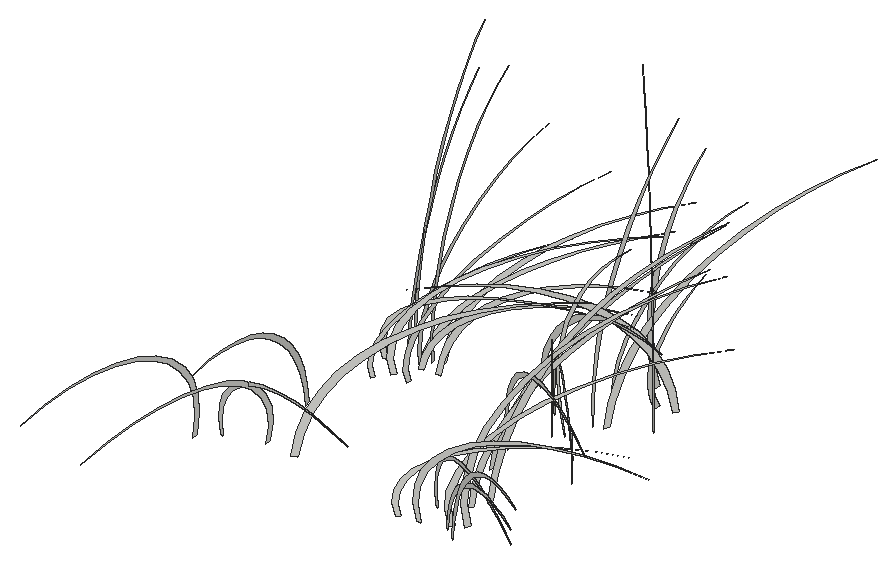
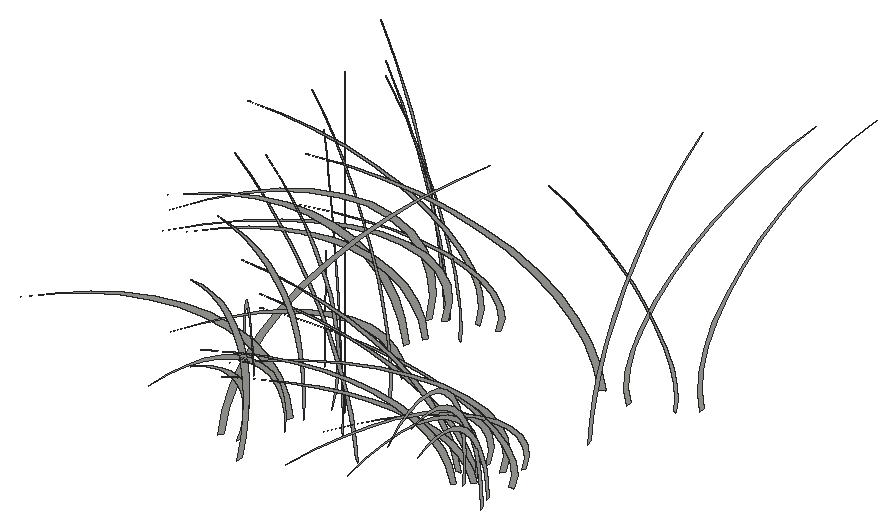
# SketchUp Ruby script. Lengths in inches.
U = 1.inch
M = Sketchup.active_model
def pt(a) = Geom::Point3d.new(a.map { |v| v * U })
def face(e, loops, mat)
  f = e.add_face(loops[0].map { |a| pt(a) })
  loops[1..].each { |l| e.add_face(l.map { |a| pt(a) }).erase! }
  f.material = f.back_material = mat if mat
  f
end
# faces: each face lists its corners as indices into pts; further lists are holes
def faces(e, pts, list, mat = nil) = list.each { |f| face(e, (f[0].is_a?(Array) ? f : [f]).map { |l| l.map { |i| pts[i] } }, mat) }
# xy, xz, yz: faces in a plane at the given z, y or x. An outline is a flat list of corners, or four numbers for a rectangle; further outlines are holes
def ring(l) = l.size == 4 ? [[l[0], l[1]], [l[2], l[1]], [l[2], l[3]], [l[0], l[3]]] : l.each_slice(2).to_a
def flat(e, list, mat, &to3) = list.each { |f| face(e, (f[0].is_a?(Array) ? f : [f]).map { |l| ring(l).map { |u, v| to3.(u, v) } }, mat) }
def xy(e, z, list, mat = nil) = flat(e, list, mat) { |x, y| [x, y, z] }
def xz(e, y, list, mat = nil) = flat(e, list, mat) { |x, z| [x, y, z] }
def yz(e, x, list, mat = nil) = flat(e, list, mat) { |y, z| [x, y, z] }
def lines(e, pts, list) = list.each { |a, b| e.add_line(pt(pts[a]), pt(pts[b])) }
# prism: a flat outline (further loops are holes) pulled along v
def prism(e, loops, v, mat = nil)
  f = face(e, loops, mat); d = Geom::Vector3d.new(v.map { |x| x * U })
  f.pushpull(f.normal.samedirection?(d) ? d.length : -d.length)
end
def box(e, o, s, mat = nil) = prism(e, [[o, [o[0] + s[0], o[1], o[2]], [o[0] + s[0], o[1] + s[1], o[2]], [o[0], o[1] + s[1], o[2]]]], [0, 0, s[2]], mat)
def at(x, y, z, deg = 0) = Geom::Transformation.translation(pt([x, y, z])) * Geom::Transformation.rotation(ORIGIN, Z_AXIS, deg.degrees)
def axes(o, x, y, z) = Geom::Transformation.new([*x, 0, *y, 0, *z, 0, *pt(o).to_a, 1])
def part(name) = M.definitions.add(name)
# library, detail: a bought-in or finely detailed component or shape, given as its bounding box
def library(name, o, s) = part(name).tap { |d| box(d.entities, o, s) }
def detail(e, o, s) = box(e.add_group.entities, o, s)
def put(e, d, t, mat = nil) = e.add_instance(d, t).tap { |i| i.material = mat if mat }
def group(e, t, mat = nil) = e.add_group.tap { |g| g.transformation = t; g.material = mat if mat }.entities
root = M.entities
g1 = group(root,at(13.87,756.7,-58.625))
p = [[0.42,-0.1875,0],[0.1875,-0.08,0],[0,0,0.76],[0.08,-0.03,1.52],[0.41,-0.18,2.27],[1,-0.45,2.98],
  [1.83,-0.82,3.65],[2.88,-1.28,4.24],[4.125,-1.84,4.76],[5.52,-2.46,5.17],[7.05,-3.14,5.49],[8.67,-3.86,5.6875],
  [10.34,-4.61,5.77],[12.01,-5.35,5.73],[10.37,-4.62,5.74],[8.74,-3.9,5.63],[7.17,-3.2,5.41],[5.69,-2.54,5.09],
  [4.33,-1.93,4.67],[3.13,-1.4,4.16],[2.11,-0.94,3.57],[1.3,-0.58,2.92],[0.72,-0.32,2.22],[0.37,-0.17,1.49],
  [0.27,-0.12,0.74]]
faces(g1,p,[[0,1,2,3,4,5,6,7,8,9,10,11,12,13,14,15,16,17,18,19,20,21,22,23,24]])
g2 = group(root,at(16.26,757.76,-58.625))
p = [[0.08,-0.6,0],[0.03,-0.27,0],[0,0,0.91],[0.01,-0.11,1.82],[0.07,-0.59,2.72],[0.18,-1.43,3.57],
  [0.33,-2.61,4.37],[0.52,-4.1,5.08],[0.74,-5.86,5.69],[0.99,-7.86,6.19],[1.26,-10.03,6.57],[1.55,-12.33,6.81],
  [1.85,-14.7,6.91],[2.15,-17.08,6.86],[1.86,-14.74,6.87],[1.57,-12.43,6.74],[1.28,-10.2,6.48],[1.02,-8.09,6.09],
  [0.78,-6.16,5.59],[0.5625,-4.45,4.98],[0.38,-3.01,4.28],[0.23,-1.85,3.5],[0.13,-1.02,2.66],[0.07,-0.53,1.79],
  [0.05,-0.39,0.89]]
faces(g2,p,[[0,1,2,3,4,5,6,7,8,9,10,11,12,13,14,15,16,17,18,19,20,21,22,23,24]])
g3 = group(root,at(17.87,768.3125,-58.625))
p = [[7.42,7.33,7.7],[8.54,8.44,7.91],[7.45,7.37,7.66],[6.41,6.33,7.32],[5.41,5.35,6.89],[4.47,4.42,6.37],
  [3.6,3.5625,5.77],[2.81,2.78,5.1],[2.12,2.09,4.37],[1.51,1.5,3.57],[1.02,1.01,2.73],[0.63,0.62,1.84],
  [0.35,0.35,0.93],[0.19,0.19,0],[0,0,0],[0.13,0.13,0.95],[0.39,0.38,1.89],[0.77,0.76,2.79],
  [1.27,1.26,3.66],[1.89,1.87,4.47],[2.61,2.58,5.21],[3.42,3.38,5.89],[4.32,4.27,6.48],[5.3,5.24,6.99],
  [6.33,6.26,7.39]]
faces(g3,p,[[0,1,2,3,4,5,6,7,8,9,10,11,12,13,14,15,16,17,18,19,20,21,22,23,24]])
g4 = group(root,at(17.79,765.61,-58.625))
p = [[0.04,0.5,0],[0.02,0.22,0],[0,0,0.75],[0.01,0.09,1.5],[0.04,0.49,2.24],[0.1,1.18,2.94],
  [0.17,2.16,3.59],[0.27,3.39,4.18],[0.39,4.85,4.6875],[0.53,6.5,5.1],[0.67,8.29,5.41],[0.82,10.19,5.6],
  [0.98,12.15,5.68],[1.14,14.12,5.64],[0.99,12.19,5.65],[0.83,10.28,5.55],[0.68,8.43,5.33],[0.54,6.69,5.02],
  [0.41,5.1,4.6],[0.3,3.68,4.1],[0.2,2.49,3.52],[0.125,1.53,2.88],[0.07,0.84,2.19],[0.04,0.4375,1.47],
  [0.03,0.32,0.73]]
faces(g4,p,[[0,1,2,3,4,5,6,7,8,9,10,11,12,13,14,15,16,17,18,19,20,21,22,23,24]])
g5 = group(root,at(16.61,765.86,-58.625))
p = [[0.33,0.33,0],[0.15,0.15,0],[0,0,0.88],[0.06,0.06,1.76],[0.32,0.32,2.63],[0.79,0.78,3.46],
  [1.43,1.42,4.23],[2.25,2.23,4.92],[3.22,3.1875,5.51],[4.32,4.27,6],[5.51,5.45,6.36],[6.77,6.7,6.59],
  [8.08,7.99,6.6875],[9.38,9.28,6.64],[8.1,8.01,6.65],[6.83,6.75,6.53],[5.6,5.54,6.28],[4.45,4.4,5.9],
  [3.39,3.35,5.41],[2.45,2.42,4.82],[1.65,1.63,4.14],[1.02,1.01,3.39],[0.5625,0.56,2.58],[0.29,0.29,1.73],
  [0.21,0.21,0.86]]
faces(g5,p,[[0,1,2,3,4,5,6,7,8,9,10,11,12,13,14,15,16,17,18,19,20,21,22,23,24]])
g6 = group(root,at(17.18,767.63,-58.625))
p = [[7.42,7.33,6.21],[8.54,8.44,6.375],[7.45,7.37,6.18],[6.41,6.33,5.9],[5.41,5.35,5.56],[4.47,4.42,5.14],
  [3.6,3.5625,4.66],[2.81,2.78,4.11],[2.12,2.09,3.52],[1.51,1.5,2.88],[1.02,1.01,2.2],[0.63,0.62,1.49],
  [0.35,0.35,0.75],[0.19,0.19,0],[0,0,0],[0.13,0.13,0.77],[0.39,0.38,1.52],[0.77,0.76,2.25],
  [1.27,1.26,2.95],[1.89,1.87,3.6],[2.61,2.58,4.21],[3.42,3.38,4.75],[4.32,4.27,5.23],[5.3,5.24,5.63],
  [6.33,6.26,5.96]]
faces(g6,p,[[0,1,2,3,4,5,6,7,8,9,10,11,12,13,14,15,16,17,18,19,20,21,22,23,24]])
g7 = group(root,at(27.74,768.2,-58.625))
p = [[4.83,11.72,10.21],[5.56,13.49,10.48],[4.85,11.77,10.15],[4.17,10.12,9.7],[3.52,8.54,9.13],[2.91,7.0625,8.44],
  [2.35,5.69,7.65],[1.83,4.45,6.76],[1.38,3.34,5.78],[0.99,2.39,4.73],[0.66,1.61,3.61],[0.41,0.99,2.44],
  [0.23,0.56,1.23],[0.125,0.31,0],[0,0,0],[0.09,0.21,1.26],[0.25,0.61,2.5],[0.5,1.22,3.7],
  [0.83,2.01,4.85],[1.23,2.98,5.92],[1.7,4.12,6.91],[2.23,5.4,7.8],[2.8125,6.83,8.59],[3.45,8.37,9.26],
  [4.125,10,9.8]]
faces(g7,p,[[0,1,2,3,4,5,6,7,8,9,10,11,12,13,14,15,16,17,18,19,20,21,22,23,24]])
g8 = group(root,at(26.19,755.85,-58.625))
p = [[0.5,0,0],[0.22,0,0],[0,0,0.95],[0.09,0,1.9],[0.49,0,2.83],[1.1875,-0.01,3.72],
  [2.17,-0.01,4.55],[3.41,-0.02,5.29],[4.87,-0.03,5.93],[6.53,-0.04,6.45],[8.33,-0.05,6.84],[10.24,-0.06,7.09],
  [12.21,-0.07,7.1875],[14.19,-0.08,7.14],[12.25,-0.07,7.15],[10.33,-0.06,7.02],[8.47,-0.05,6.75],[6.72,-0.04,6.35],
  [5.12,-0.03,5.82],[3.7,-0.02,5.18],[2.5,-0.01,4.45],[1.54,-0.01,3.64],[0.85,0,2.77],[0.44,0,1.86],
  [0.32,0,0.93]]
faces(g8,p,[[0,1,2,3,4,5,6,7,8,9,10,11,12,13,14,15,16,17,18,19,20,21,22,23,24]])
g9 = group(root,at(17.96,757.02,-58.625))
p = [[11.7,4.87,10.21],[13.47,5.61,10.48],[11.76,4.89,10.15],[10.11,4.21,9.7],[8.53,3.55,9.13],[7.05,2.94,8.44],
  [5.68,2.37,7.65],[4.44,1.85,6.76],[3.34,1.39,5.78],[2.39,0.99,4.73],[1.6,0.67,3.61],[0.99,0.41,2.44],
  [0.56,0.23,1.23],[0.3,0.125,0],[0,0,0],[0.21,0.09,1.26],[0.61,0.26,2.5],[1.22,0.51,3.7],
  [2.01,0.84,4.85],[2.98,1.24,5.92],[4.11,1.71,6.91],[5.4,2.25,7.8],[6.82,2.84,8.59],[8.36,3.48,9.26],
  [9.99,4.16,9.8]]
faces(g9,p,[[0,1,2,3,4,5,6,7,8,9,10,11,12,13,14,15,16,17,18,19,20,21,22,23,24]])
g10 = group(root,at(15.5,769.27,-58.625))
p = [[-4.01,9.63,10.42],[-4.61,11.08,10.69],[-4.03,9.68,10.36],[-3.46,8.32,9.9],[-2.92,7.02,9.32],[-2.42,5.8,8.62],
  [-1.95,4.68,7.81],[-1.52,3.65,6.9],[-1.14,2.75,5.9],[-0.82,1.97,4.83],[-0.55,1.32,3.6875],[-0.34,0.81,2.49],
  [-0.19,0.46,1.26],[-0.1,0.25,0],[0,0,0],[-0.07,0.17,1.29],[-0.21,0.5,2.55],[-0.42,1,3.78],
  [-0.6875,1.65,4.95],[-1.02,2.45,6.04],[-1.41,3.38,7.05],[-1.85,4.44,7.96],[-2.34,5.61,8.76],[-2.86,6.875,9.45],
  [-3.42,8.22,10]]
faces(g10,p,[[0,1,2,3,4,5,6,7,8,9,10,11,12,13,14,15,16,17,18,19,20,21,22,23,24]])
g11 = group(root,at(17.67,767.86,-58.625))
p = [[-0.18,0.43,0],[-0.08,0.19,0],[0,0,1.1875],[-0.03,0.08,2.38],[-0.17,0.42,3.56],[-0.42,1.02,4.68],
  [-0.77,1.86,5.72],[-1.22,2.92,6.65],[-1.74,4.18,7.45],[-2.33,5.6,8.11],[-2.98,7.16,8.6],[-3.66,8.8,8.91],
  [-4.36,10.49,9.04],[-5.07,12.18,8.98],[-4.38,10.52,8.99],[-3.69,8.87,8.83],[-3.03,7.28,8.49],[-2.4,5.77,7.98],
  [-1.83,4.4,7.32],[-1.32,3.18,6.52],[-0.89,2.15,5.6],[-0.55,1.32,4.58],[-0.3,0.73,3.48],[-0.16,0.38,2.34],
  [-0.12,0.28,1.17]]
faces(g11,p,[[0,1,2,3,4,5,6,7,8,9,10,11,12,13,14,15,16,17,18,19,20,21,22,23,24]])
g12 = group(root,at(17.43,767.15,-58.625))
p = [[-0.09,0.46,0],[-0.04,0.2,0],[0,0,0.88],[-0.02,0.08,1.76],[-0.09,0.45,2.63],[-0.21,1.08,3.46],
  [-0.38,1.98,4.23],[-0.6,3.11,4.92],[-0.86,4.45,5.51],[-1.16,5.96,6],[-1.48,7.61,6.36],[-1.8125,9.35,6.59],
  [-2.16,11.15,6.6875],[-2.51,12.96,6.64],[-2.17,11.18,6.65],[-1.83,9.43,6.53],[-1.5,7.74,6.28],[-1.19,6.14,5.9],
  [-0.91,4.67,5.41],[-0.66,3.38,4.82],[-0.44,2.28,4.14],[-0.27,1.41,3.39],[-0.15,0.77,2.58],[-0.08,0.4,1.73],
  [-0.06,0.29,0.86]]
faces(g12,p,[[0,1,2,3,4,5,6,7,8,9,10,11,12,13,14,15,16,17,18,19,20,21,22,23,24]])
g13 = group(root,at(15.87,768.38,-58.625))
p = [[-4.01,9.63,8.4],[-4.61,11.08,8.62],[-4.03,9.68,8.35],[-3.46,8.32,7.98],[-2.92,7.02,7.51],[-2.42,5.8,6.95],
  [-1.95,4.68,6.3],[-1.52,3.65,5.5625],[-1.14,2.75,4.76],[-0.82,1.97,3.89],[-0.55,1.32,2.97],[-0.34,0.81,2.01],
  [-0.19,0.46,1.02],[-0.1,0.25,0],[0,0,0],[-0.07,0.17,1.04],[-0.21,0.5,2.06],[-0.42,1,3.05],
  [-0.6875,1.65,3.99],[-1.02,2.45,4.87],[-1.41,3.38,5.6875],[-1.85,4.44,6.42],[-2.34,5.61,7.07],[-2.86,6.875,7.62],
  [-3.42,8.22,8.0625]]
faces(g13,p,[[0,1,2,3,4,5,6,7,8,9,10,11,12,13,14,15,16,17,18,19,20,21,22,23,24]])
g14 = group(root,at(25.05,764.17,-58.625))
p = [[0.45,-0.35,0],[0.2,-0.15,0],[0,0,1.07],[0.08,-0.0625,2.14],[0.4375,-0.34,3.2],[1.06,-0.82,4.2],
  [1.94,-1.5,5.14],[3.04,-2.36,5.98],[4.35,-3.375,6.7],[5.83,-4.52,7.29],[7.4375,-5.77,7.73],[9.14,-7.1,8.01],
  [10.9,-8.46,8.125],[12.67,-9.83,8.07],[10.93,-8.49,8.08],[9.22,-7.16,7.93],[7.5625,-5.87,7.625],[6,-4.66,7.17],
  [4.57,-3.55,6.58],[3.3,-2.56,5.86],[2.23,-1.73,5.03],[1.375,-1.07,4.12],[0.76,-0.59,3.13],[0.39,-0.3,2.1],
  [0.29,-0.22,1.05]]
faces(g14,p,[[0,1,2,3,4,5,6,7,8,9,10,11,12,13,14,15,16,17,18,19,20,21,22,23,24]])
g15 = group(root,at(22.73,769.59,-58.625))
p = [[11.19,-5.95,8.88],[12.88,-6.85,9.11],[11.24,-5.98,8.83],[9.66,-5.14,8.4375],[8.16,-4.34,7.94],[6.74,-3.59,7.34],
  [5.43,-2.89,6.66],[4.25,-2.26,5.88],[3.19,-1.7,5.03],[2.29,-1.22,4.12],[1.53,-0.82,3.14],[0.95,-0.5,2.125],
  [0.53,-0.28,1.07],[0.29,-0.16,0],[0,0,0],[0.2,-0.1,1.1],[0.59,-0.3125,2.18],[1.16,-0.62,3.22],
  [1.92,-1.02,4.22],[2.85,-1.51,5.15],[3.93,-2.09,6.01],[5.16,-2.74,6.79],[6.52,-3.47,7.47],[7.99,-4.25,8.05],
  [9.55,-5.08,8.52]]
faces(g15,p,[[0,1,2,3,4,5,6,7,8,9,10,11,12,13,14,15,16,17,18,19,20,21,22,23,24]])
g16 = group(root,at(27.9375,759.28,-58.625))
p = [[4.27,10.37,11.2],[4.92,11.93,11.5],[4.29,10.42,11.14],[3.69,8.96,10.64],[3.12,7.56,10.02],[2.58,6.25,9.26],
  [2.08,5.04,8.4],[1.62,3.94,7.42],[1.22,2.96,6.35],[0.87,2.12,5.19],[0.59,1.42,3.97],[0.36,0.88,2.68],
  [0.2,0.49,1.35],[0.11,0.27,0],[0,0,0],[0.08,0.18,1.39],[0.22,0.54,2.75],[0.44,1.08,4.0625],
  [0.73,1.78,5.32],[1.09,2.64,6.5],[1.5,3.64,7.58],[1.97,4.78,8.5625],[2.49,6.04,9.42],[3.05,7.4,10.16],
  [3.65,8.85,10.75]]
faces(g16,p,[[0,1,2,3,4,5,6,7,8,9,10,11,12,13,14,15,16,17,18,19,20,21,22,23,24]])
g17 = group(root,at(28.51,756.56,-58.625))
p = [[0.19,0.46,0],[0.08,0.21,0],[0,0,1.28],[0.03,0.08,2.5625],[0.1875,0.45,3.82],[0.45,1.1,5.03],
  [0.83,2,6.15],[1.3,3.15,7.15],[1.86,4.5,8.02],[2.49,6.04,8.72],[3.18,7.7,9.25],[3.9,9.47,9.58],
  [4.65,11.29,9.72],[5.41,13.12,9.66],[4.67,11.33,9.67],[3.9375,9.55,9.49],[3.23,7.83,9.125],[2.5625,6.22,8.58],
  [1.95,4.73,7.87],[1.41,3.42,7.01],[0.95,2.31,6.02],[0.59,1.42,4.92],[0.32,0.78,3.75],[0.17,0.41,2.51],
  [0.12,0.3,1.26]]
faces(g17,p,[[0,1,2,3,4,5,6,7,8,9,10,11,12,13,14,15,16,17,18,19,20,21,22,23,24]])
g18 = group(root,at(27.8,756.2,-58.625))
p = [[0.28,0.41,0],[0.125,0.18,0],[0,0,0.95],[0.05,0.07,1.9],[0.27,0.41,2.83],[0.66,0.98,3.72],
  [1.21,1.8,4.55],[1.91,2.82,5.29],[2.73,4.04,5.93],[3.65,5.41,6.45],[4.66,6.91,6.84],[5.73,8.49,7.09],
  [6.83,10.12,7.1875],[7.9375,11.76,7.14],[6.85,10.15,7.15],[5.78,8.5625,7.02],[4.74,7.02,6.75],[3.76,5.57,6.35],
  [2.86,4.24,5.82],[2.07,3.07,5.18],[1.4,2.07,4.45],[0.86,1.28,3.64],[0.47,0.7,2.77],[0.25,0.36,1.86],
  [0.18,0.27,0.93]]
faces(g18,p,[[0,1,2,3,4,5,6,7,8,9,10,11,12,13,14,15,16,17,18,19,20,21,22,23,24]])
g19 = group(root,at(28.67,755.65,-58.625))
p = [[8.86,-6.88,8.28],[10.2,-7.92,8.5],[8.9,-6.91,8.24],[7.65,-5.94,7.87],[6.46,-5.01,7.41],[5.34,-4.14,6.85],
  [4.3,-3.34,6.21],[3.36,-2.61,5.49],[2.53,-1.96,4.69],[1.81,-1.4,3.84],[1.21,-0.94,2.93],[0.75,-0.58,1.98],
  [0.42,-0.33,1],[0.23,-0.18,0],[0,0,0],[0.16,-0.12,1.03],[0.46,-0.36,2.03],[0.92,-0.71,3],
  [1.52,-1.18,3.93],[2.25,-1.75,4.8],[3.11,-2.42,5.61],[4.09,-3.17,6.33],[5.16,-4.01,6.97],[6.33,-4.91,7.51],
  [7.5625,-5.87,7.95]]
faces(g19,p,[[0,1,2,3,4,5,6,7,8,9,10,11,12,13,14,15,16,17,18,19,20,21,22,23,24]])
g20 = group(root,at(27.54,758.32,-58.625))
p = [[4.27,10.37,9.03],[4.92,11.93,9.27],[4.29,10.42,8.98],[3.69,8.96,8.58],[3.12,7.56,8.08],[2.58,6.25,7.47],
  [2.08,5.04,6.77],[1.62,3.94,5.98],[1.22,2.96,5.12],[0.87,2.12,4.1875],[0.59,1.42,3.2],[0.36,0.88,2.16],
  [0.2,0.49,1.09],[0.11,0.27,0],[0,0,0],[0.08,0.18,1.12],[0.22,0.54,2.22],[0.44,1.08,3.28],
  [0.73,1.78,4.29],[1.09,2.64,5.24],[1.5,3.64,6.11],[1.97,4.78,6.9],[2.49,6.04,7.6],[3.05,7.4,8.19],
  [3.65,8.85,8.67]]
faces(g20,p,[[0,1,2,3,4,5,6,7,8,9,10,11,12,13,14,15,16,17,18,19,20,21,22,23,24]])
g21 = group(root,at(13.21,756.0625,-58.625))
p = [[0.07,-0.56,0],[0.03,-0.25,0],[0,0,1.07],[0.01,-0.1,2.14],[0.07,-0.55,3.2],[0.17,-1.33,4.2],
  [0.31,-2.43,5.14],[0.48,-3.82,5.98],[0.6875,-5.46,6.7],[0.92,-7.32,7.29],[1.18,-9.34,7.73],[1.45,-11.49,8.01],
  [1.72,-13.69,8.125],[2,-15.91,8.07],[1.73,-13.73,8.08],[1.46,-11.58,7.93],[1.2,-9.5,7.625],[0.95,-7.54,7.17],
  [0.72,-5.74,6.58],[0.52,-4.15,5.86],[0.35,-2.8,5.03],[0.22,-1.73,4.12],[0.12,-0.95,3.13],[0.0625,-0.49,2.1],
  [0.05,-0.36,1.05]]
faces(g21,p,[[0,1,2,3,4,5,6,7,8,9,10,11,12,13,14,15,16,17,18,19,20,21,22,23,24]])
g22 = group(root,at(15.4,761.53,-58.625))
p = [[3.71,-12.12,8.88],[4.26,-13.95,9.11],[3.72,-12.18,8.83],[3.2,-10.47,8.4375],[2.7,-8.84,7.94],[2.23,-7.3,7.34],
  [1.8,-5.89,6.66],[1.41,-4.6,5.88],[1.06,-3.46,5.03],[0.76,-2.48,4.12],[0.51,-1.66,3.14],[0.3125,-1.03,2.125],
  [0.18,-0.58,1.07],[0.1,-0.32,0],[0,0,0],[0.07,-0.21,1.1],[0.19,-0.64,2.18],[0.39,-1.26,3.22],
  [0.64,-2.08,4.22],[0.94,-3.08,5.15],[1.3,-4.26,6.01],[1.71,-5.59,6.79],[2.16,-7.0625,7.47],[2.65,-8.65,8.05],
  [3.16,-10.35,8.52]]
faces(g22,p,[[0,1,2,3,4,5,6,7,8,9,10,11,12,13,14,15,16,17,18,19,20,21,22,23,24]])
g23 = group(root,at(18.37,767.36,-58.625))
p = [[10.35,1.3,7.7],[11.91,1.5,7.91],[10.4,1.31,7.66],[8.9375,1.125,7.32],[7.55,0.95,6.89],[6.24,0.79,6.37],
  [5.03,0.63,5.77],[3.93,0.49,5.1],[2.95,0.37,4.37],[2.11,0.27,3.57],[1.42,0.18,2.73],[0.875,0.11,1.84],
  [0.49,0.0625,0.93],[0.27,0.03,0],[0,0,0],[0.18,0.02,0.95],[0.54,0.07,1.89],[1.08,0.14,2.79],
  [1.78,0.22,3.66],[2.63,0.33,4.47],[3.64,0.46,5.21],[4.77,0.6,5.89],[6.03,0.76,6.48],[7.39,0.93,6.99],
  [8.84,1.11,7.39]]
faces(g23,p,[[0,1,2,3,4,5,6,7,8,9,10,11,12,13,14,15,16,17,18,19,20,21,22,23,24]])
g24 = group(root,at(17.41,767.24,-58.625))
p = [[10.35,1.3,6.21],[11.91,1.5,6.375],[10.4,1.31,6.18],[8.9375,1.125,5.9],[7.55,0.95,5.56],[6.24,0.79,5.14],
  [5.03,0.63,4.66],[3.93,0.49,4.11],[2.95,0.37,3.52],[2.11,0.27,2.88],[1.42,0.18,2.2],[0.875,0.11,1.49],
  [0.49,0.0625,0.75],[0.27,0.03,0],[0,0,0],[0.18,0.02,0.77],[0.54,0.07,1.52],[1.08,0.14,2.25],
  [1.78,0.22,2.95],[2.63,0.33,3.6],[3.64,0.46,4.21],[4.77,0.6,4.75],[6.03,0.76,5.23],[7.39,0.93,5.63],
  [8.84,1.11,5.96]]
faces(g24,p,[[0,1,2,3,4,5,6,7,8,9,10,11,12,13,14,15,16,17,18,19,20,21,22,23,24]])
g25 = group(root,at(16.13,765.01,-58.625))
p = [[0.16,0.35,0],[0.07,0.15,0],[0,0,0.625],[0.03,0.0625,1.25],[0.15,0.34,1.87],[0.37,0.83,2.46],
  [0.67,1.51,3],[1.06,2.37,3.49],[1.51,3.39,3.91],[2.03,4.55,4.26],[2.59,5.8,4.52],[3.18,7.14,4.68],
  [3.79,8.51,4.75],[4.41,9.88,4.72],[3.8,8.53,4.72],[3.21,7.2,4.63],[2.63,5.9,4.46],[2.09,4.68,4.19],
  [1.59,3.57,3.84],[1.15,2.58,3.42],[0.78,1.74,2.94],[0.48,1.07,2.4],[0.26,0.59,1.83],[0.14,0.31,1.23],
  [0.1,0.22,0.61]]
faces(g25,p,[[0,1,2,3,4,5,6,7,8,9,10,11,12,13,14,15,16,17,18,19,20,21,22,23,24]])
g26 = group(root,at(15.26,766.97,-58.625))
p = [[0.49,0.0625,0],[0.22,0.03,0],[0,0,0.75],[0.09,0.01,1.5],[0.48,0.0625,2.24],[1.18,0.15,2.94],
  [2.15,0.27,3.59],[3.375,0.42,4.18],[4.83,0.61,4.6875],[6.47,0.8125,5.1],[8.25,1.04,5.41],[10.15,1.28,5.6],
  [12.1,1.52,5.68],[14.06,1.77,5.64],[12.13,1.53,5.65],[10.23,1.29,5.55],[8.39,1.06,5.33],[6.66,0.84,5.02],
  [5.07,0.64,4.6],[3.67,0.46,4.1],[2.48,0.3125,3.52],[1.53,0.19,2.88],[0.84,0.11,2.19],[0.44,0.05,1.47],
  [0.32,0.04,0.73]]
faces(g26,p,[[0,1,2,3,4,5,6,7,8,9,10,11,12,13,14,15,16,17,18,19,20,21,22,23,24]])
g27 = group(root,at(27.26,767.95,-58.625))
yz(g27,0,[[0.08,0,0,1.22,0.03,2.45,0.18,3.67,0.44,4.88,0.82,6.08,1.31,7.26,1.91,8.42,2.62,9.56,3.43,10.66,4.35,11.73,5.37,12.76,6.48,13.75,5.44,12.74,4.5,11.6875,3.63,10.61,2.86,9.5,2.18,8.36,1.59,7.21,1.09,6.03,0.7,4.84,0.4,3.64,0.19,2.43,0.09,1.22]])
g28 = group(root,at(24.75,768.21,-58.625))
p = [[0.4,-0.45,0],[0.18,-0.2,0],[0,0,0.91],[0.07,-0.08,1.82],[0.39,-0.44,2.72],[0.96,-1.08,3.57],
  [1.75,-1.97,4.37],[2.74,-3.09,5.08],[3.92,-4.42,5.69],[5.26,-5.92,6.19],[6.71,-7.5625,6.57],[8.25,-9.3,6.81],
  [9.83,-11.08,6.91],[11.42,-12.875,6.86],[9.86,-11.12,6.87],[8.32,-9.375,6.74],[6.82,-7.6875,6.48],[5.41,-6.1,6.09],
  [4.12,-4.65,5.59],[2.98,-3.36,4.98],[2.01,-2.27,4.28],[1.24,-1.4,3.5],[0.68,-0.77,2.66],[0.35,-0.4,1.79],
  [0.26,-0.29,0.89]]
faces(g28,p,[[0,1,2,3,4,5,6,7,8,9,10,11,12,13,14,15,16,17,18,19,20,21,22,23,24]])
g29 = group(root,at(29.31,763.87,-58.625))
p = [[2.68,-3.47,4.09],[2.1875,-2.83,3.83],[1.75,-2.26,3.54],[1.35,-1.75,3.24],[1.02,-1.32,2.91],[0.74,-0.96,2.57],
  [0.52,-0.68,2.22],[0.37,-0.48,1.85],[0.28,-0.36,1.48],[0.25,-0.33,1.11],[0.29,-0.375,0.73],[0.39,-0.51,0.36],
  [0.56,-0.73,0],[0.34,-0.45,0],[0.16,-0.21,0.37],[0.04,-0.06,0.74],[0,0,1.125],[0.03,-0.04,1.51],
  [0.13,-0.17,1.88],[0.3,-0.39,2.25],[0.55,-0.71,2.61],[0.85,-1.11,2.95],[1.23,-1.59,3.27],[1.66,-2.15,3.57],
  [2.14,-2.77,3.84]]
faces(g29,p,[[0,1,2,3,4,5,6,7,8,9,10,11,12,13,14,15,16,17,18,19,20,21,22,23,24]])
g30 = group(root,at(29.49,771.68,-58.625))
p = [[-4.83,-11.72,10.21],[-5.56,-13.49,10.48],[-4.85,-11.77,10.15],[-4.17,-10.12,9.7],[-3.52,-8.54,9.13],[-2.91,-7.0625,8.44],
  [-2.35,-5.69,7.65],[-1.83,-4.45,6.76],[-1.38,-3.34,5.78],[-0.99,-2.39,4.73],[-0.66,-1.61,3.61],[-0.41,-0.99,2.44],
  [-0.23,-0.56,1.23],[-0.125,-0.31,0],[0,0,0],[-0.09,-0.21,1.26],[-0.25,-0.61,2.5],[-0.5,-1.22,3.7],
  [-0.83,-2.01,4.85],[-1.23,-2.98,5.92],[-1.7,-4.12,6.91],[-2.23,-5.4,7.8],[-2.8125,-6.83,8.59],[-3.45,-8.37,9.26],
  [-4.125,-10,9.8]]
faces(g30,p,[[0,1,2,3,4,5,6,7,8,9,10,11,12,13,14,15,16,17,18,19,20,21,22,23,24]])
g31 = group(root,at(26.26,766.54,-58.625))
p = [[0.57,-0.08,0],[0.26,-0.04,1.02],[0.0625,-0.01,2.05],[0,0,3.09],[0.0625,-0.01,4.12],[0.25,-0.04,5.15],
  [0.57,-0.08,6.17],[1.01,-0.15,7.18],[1.57,-0.23,8.17],[2.25,-0.33,9.14],[3.05,-0.44,10.08],[3.97,-0.57,10.99],
  [4.99,-0.72,11.87],[4.03,-0.58,10.98],[3.16,-0.46,10.06],[2.41,-0.35,9.11],[1.75,-0.25,8.14],[1.21,-0.18,7.16],
  [0.78,-0.11,6.15],[0.46,-0.07,5.14],[0.25,-0.04,4.11],[0.16,-0.02,3.08],[0.18,-0.03,2.05],[0.32,-0.05,1.02]]
faces(g31,p,[[0,1,2,3,4,5,6,7,8,9,10,11,12,13,14,15,16,17,18,19,20,21,22,23]])
g32 = group(root,at(28.4375,770.62,-58.625))
yz(g32,0,[[0.5625,0,0.26,0.5,0.07,1.01,0,1.52,0.05,2.04,0.21,2.55,0.5,3.05,0.89,3.53,1.4,3.99,2.01,4.43,2.71,4.83,3.51,5.2,4.38,5.53,3.58,5.18,2.86,4.79,2.22,4.38,1.67,3.9375,1.21,3.48,0.86,3,0.6,2.5,0.45,2,0.41,1.5,0.47,0.99,0.64,0.49,0.92,0]])
g33 = group(root,at(27.26,769.34,-58.625))
yz(g33,0,[[0.09,0,0,0.91,0.12,1.83,0.45,2.72,0.98,3.57,1.7,4.35,2.59,5.0625,3.64,5.68,4.81,6.18,6.09,6.57,7.44,6.83,8.84,6.95,10.25,6.9375,8.87,6.89,7.51,6.73,6.21,6.4375,4.97,6.04,3.84,5.53,2.82,4.92,1.94,4.23,1.22,3.47,0.66,2.65,0.28,1.78,0.09,0.9]])
g34 = group(root,at(27.26,772.09,-58.625))
yz(g34,0,[[0.5625,0,0.26,1.01,0.07,2.04,0,3.09,0.05,4.14,0.21,5.18,0.5,6.19,0.89,7.17,1.4,8.11,2.01,9,2.71,9.82,3.51,10.57,4.38,11.24,3.58,10.52,2.86,9.74,2.22,8.9,1.67,8,1.21,7.07,0.86,6.09,0.6,5.09,0.45,4.07,0.41,3.04,0.47,2.01,0.64,1,0.92,0]])
g35 = group(root,at(26.04,761.79,-58.625))
p = [[2.36,12.45,7.55],[2.71,14.33,7.75],[2.37,12.51,7.51],[2.04,10.75,7.17],[1.72,9.08,6.75],[1.42,7.5,6.24],
  [1.15,6.05,5.66],[0.89,4.73,5],[0.67,3.55,4.28],[0.48,2.54,3.5],[0.32,1.71,2.67],[0.2,1.05,1.81],
  [0.11,0.59,0.91],[0.0625,0.32,0],[0,0,0],[0.04,0.22,0.93],[0.125,0.65,1.85],[0.25,1.29,2.74],
  [0.4,2.14,3.58],[0.6,3.17,4.38],[0.83,4.375,5.11],[1.09,5.74,5.77],[1.375,7.26,6.35],[1.68,8.89,6.85],
  [2.01,10.63,7.25]]
faces(g35,p,[[0,1,2,3,4,5,6,7,8,9,10,11,12,13,14,15,16,17,18,19,20,21,22,23,24]])
g36 = group(root,at(25.98,766.5,-58.625))
p = [[0.35,-0.44,0],[0.16,-0.2,0],[0,0,1.26],[0.0625,-0.08,2.52],[0.35,-0.43,3.76],[0.84,-1.05,4.94],
  [1.53,-1.91,6.04],[2.41,-3,7.03],[3.44,-4.3,7.88],[4.61,-5.76,8.57],[5.89,-7.35,9.09],[7.24,-9.03,9.42],
  [8.63,-10.77,9.56],[10.03,-12.51,9.49],[8.66,-10.8,9.51],[7.3,-9.11,9.33],[5.99,-7.47,8.97],[4.75,-5.93,8.44],
  [3.62,-4.52,7.74],[2.61,-3.26,6.89],[1.77,-2.2,5.92],[1.09,-1.36,4.84],[0.6,-0.75,3.68],[0.3125,-0.39,2.47],
  [0.23,-0.28,1.23]]
faces(g36,p,[[0,1,2,3,4,5,6,7,8,9,10,11,12,13,14,15,16,17,18,19,20,21,22,23,24]])
g37 = group(root,at(25.98,766.5,-58.625))
p = [[0.35,-0.44,0],[0.16,-0.2,0],[0,0,1.26],[0.0625,-0.08,2.52],[0.35,-0.43,3.76],[0.84,-1.05,4.94],
  [1.53,-1.91,6.04],[2.41,-3,7.03],[3.44,-4.3,7.88],[4.61,-5.76,8.57],[5.89,-7.35,9.09],[7.24,-9.03,9.42],
  [8.63,-10.77,9.56],[10.03,-12.51,9.49],[8.66,-10.8,9.51],[7.3,-9.11,9.33],[5.99,-7.47,8.97],[4.75,-5.93,8.44],
  [3.62,-4.52,7.74],[2.61,-3.26,6.89],[1.77,-2.2,5.92],[1.09,-1.36,4.84],[0.6,-0.75,3.68],[0.3125,-0.39,2.47],
  [0.23,-0.28,1.23]]
faces(g37,p,[[0,1,2,3,4,5,6,7,8,9,10,11,12,13,14,15,16,17,18,19,20,21,22,23,24]])
g38 = group(root,at(29.98,769.14,-58.625))
p = [[-0.37,0.43,0],[-0.16,0.19,0],[0,0,1.44],[-0.07,0.08,2.9],[-0.36,0.42,4.32],[-0.87,1.02,5.68],
  [-1.59,1.86,6.95],[-2.5,2.93,8.08],[-3.58,4.1875,9.06],[-4.79,5.61,9.85],[-6.12,7.16,10.45],[-7.52,8.8,10.83],
  [-8.96,10.49,10.99],[-10.41,12.19,10.91],[-8.99,10.53,10.93],[-7.58,8.875,10.72],[-6.22,7.28,10.3125],[-4.93,5.78,9.7],
  [-3.76,4.4,8.89],[-2.72,3.18,7.92],[-1.83,2.15,6.8],[-1.13,1.32,5.57],[-0.62,0.73,4.23],[-0.32,0.38,2.84],
  [-0.24,0.28,1.42]]
faces(g38,p,[[0,1,2,3,4,5,6,7,8,9,10,11,12,13,14,15,16,17,18,19,20,21,22,23,24]])
g39 = group(root,at(27.85,756.29,-58.625))
p = [[8.86,-6.88,6.68],[10.2,-7.92,6.86],[8.9,-6.91,6.64],[7.65,-5.94,6.35],[6.46,-5.01,5.97],[5.34,-4.14,5.52],
  [4.3,-3.34,5.01],[3.36,-2.61,4.42],[2.53,-1.96,3.79],[1.81,-1.4,3.1],[1.21,-0.94,2.36],[0.75,-0.58,1.6],
  [0.42,-0.33,0.81],[0.23,-0.18,0],[0,0,0],[0.16,-0.12,0.83],[0.46,-0.36,1.64],[0.92,-0.71,2.42],
  [1.52,-1.18,3.17],[2.25,-1.75,3.875],[3.11,-2.42,4.52],[4.09,-3.17,5.11],[5.16,-4.01,5.62],[6.33,-4.91,6.06],
  [7.5625,-5.87,6.41]]
faces(g39,p,[[0,1,2,3,4,5,6,7,8,9,10,11,12,13,14,15,16,17,18,19,20,21,22,23,24]])
g40 = group(root,at(25.18,755.5625,-58.625))
p = [[0.38,0.15,0],[0.17,0.07,0],[0,0,0.67],[0.07,0.03,1.35],[0.375,0.14,2.01],[0.91,0.35,2.64],
  [1.66,0.64,3.23],[2.61,1,3.75],[3.73,1.43,4.21],[5,1.92,4.58],[6.38,2.45,4.86],[7.84,3.01,5.03],
  [9.35,3.59,5.1],[10.86,4.17,5.07],[9.38,3.6,5.08],[7.91,3.03,4.98],[6.49,2.49,4.79],[5.15,1.97,4.51],
  [3.92,1.5,4.13],[2.83,1.09,3.68],[1.91,0.73,3.16],[1.18,0.45,2.59],[0.65,0.25,1.97],[0.34,0.13,1.32],
  [0.25,0.09,0.66]]
faces(g40,p,[[0,1,2,3,4,5,6,7,8,9,10,11,12,13,14,15,16,17,18,19,20,21,22,23,24]])
g41 = group(root,at(26.01,757.72,-58.625))
p = [[0.42,-0.33,0],[0.1875,-0.15,0],[0,0,0.8],[0.08,-0.06,1.61],[0.41,-0.32,2.4],[1.01,-0.78,3.16],
  [1.84,-1.43,3.86],[2.89,-2.24,4.49],[4.13,-3.21,5.04],[5.54,-4.3,5.48],[7.07,-5.49,5.8125],[8.6875,-6.74,6.02],
  [10.36,-8.04,6.11],[12.03,-9.34,6.07],[10.39,-8.0625,6.08],[8.76,-6.8,5.97],[7.19,-5.58,5.74],[5.7,-4.43,5.39],
  [4.34,-3.37,4.95],[3.14,-2.4375,4.41],[2.12,-1.64,3.78],[1.31,-1.01,3.1],[0.72,-0.56,2.36],[0.37,-0.29,1.58],
  [0.27,-0.21,0.79]]
faces(g41,p,[[0,1,2,3,4,5,6,7,8,9,10,11,12,13,14,15,16,17,18,19,20,21,22,23,24]])
